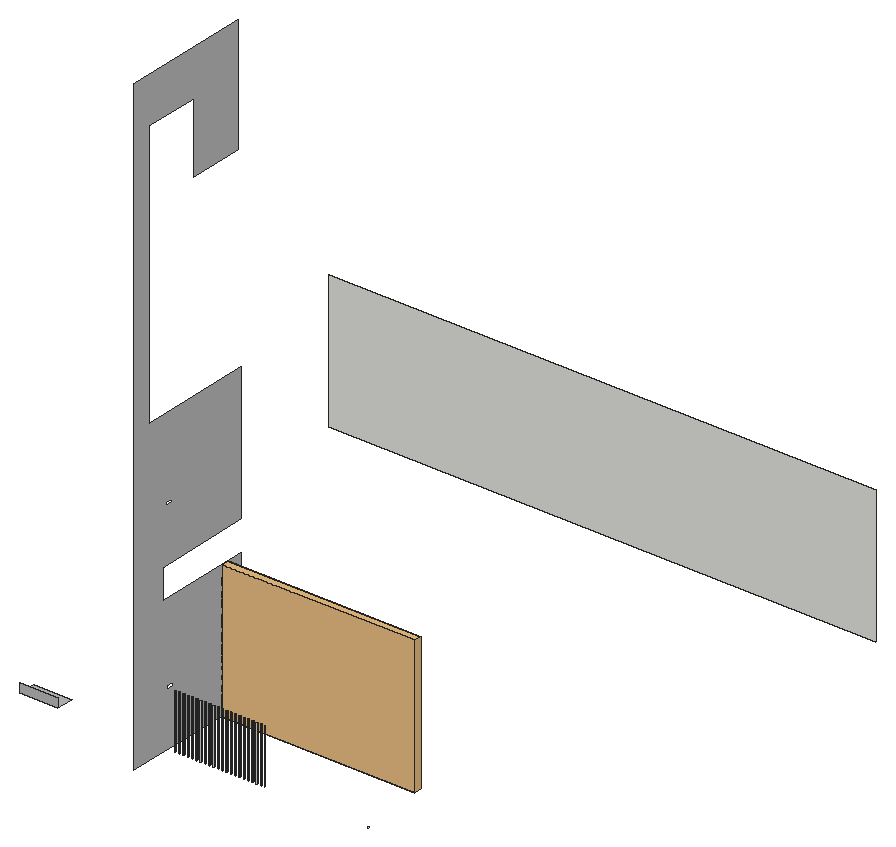
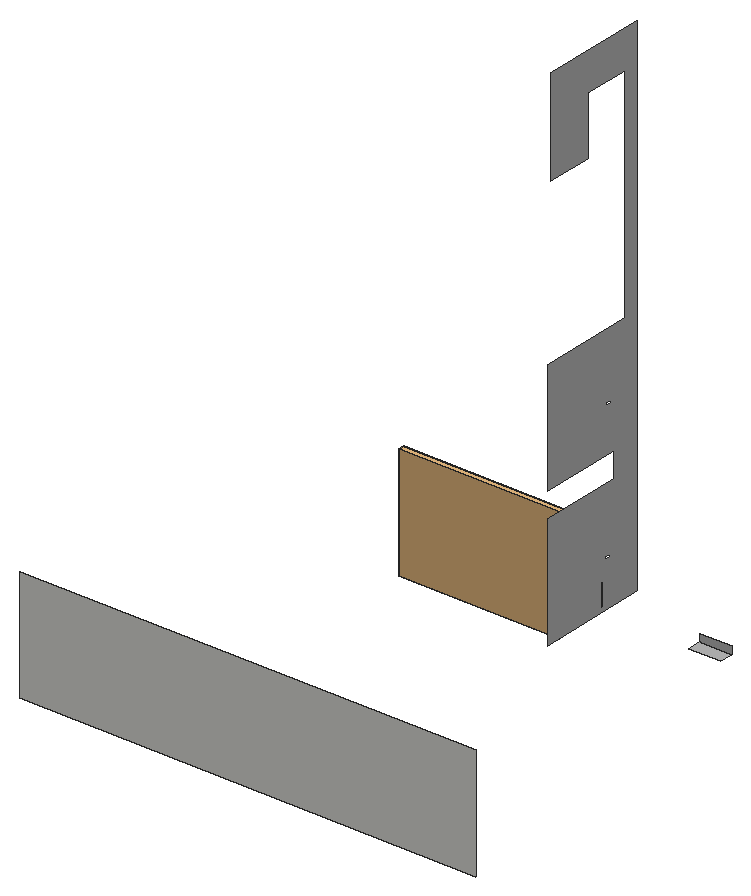
# SketchUp Ruby script. Lengths in inches.
U = 1.inch
M = Sketchup.active_model
def pt(a) = Geom::Point3d.new(a.map { |v| v * U })
def face(e, loops, mat)
  f = e.add_face(loops[0].map { |a| pt(a) })
  loops[1..].each { |l| e.add_face(l.map { |a| pt(a) }).erase! }
  f.material = f.back_material = mat if mat
  f
end
# faces: each face lists its corners as indices into pts; further lists are holes
def faces(e, pts, list, mat = nil) = list.each { |f| face(e, (f[0].is_a?(Array) ? f : [f]).map { |l| l.map { |i| pts[i] } }, mat) }
# xy, xz, yz: faces in a plane at the given z, y or x. An outline is a flat list of corners, or four numbers for a rectangle; further outlines are holes
def ring(l) = l.size == 4 ? [[l[0], l[1]], [l[2], l[1]], [l[2], l[3]], [l[0], l[3]]] : l.each_slice(2).to_a
def flat(e, list, mat, &to3) = list.each { |f| face(e, (f[0].is_a?(Array) ? f : [f]).map { |l| ring(l).map { |u, v| to3.(u, v) } }, mat) }
def xy(e, z, list, mat = nil) = flat(e, list, mat) { |x, y| [x, y, z] }
def xz(e, y, list, mat = nil) = flat(e, list, mat) { |x, z| [x, y, z] }
def yz(e, x, list, mat = nil) = flat(e, list, mat) { |y, z| [x, y, z] }
def lines(e, pts, list) = list.each { |a, b| e.add_line(pt(pts[a]), pt(pts[b])) }
# prism: a flat outline (further loops are holes) pulled along v
def prism(e, loops, v, mat = nil)
  f = face(e, loops, mat); d = Geom::Vector3d.new(v.map { |x| x * U })
  f.pushpull(f.normal.samedirection?(d) ? d.length : -d.length)
end
def box(e, o, s, mat = nil) = prism(e, [[o, [o[0] + s[0], o[1], o[2]], [o[0] + s[0], o[1] + s[1], o[2]], [o[0], o[1] + s[1], o[2]]]], [0, 0, s[2]], mat)
def at(x, y, z, deg = 0) = Geom::Transformation.translation(pt([x, y, z])) * Geom::Transformation.rotation(ORIGIN, Z_AXIS, deg.degrees)
def axes(o, x, y, z) = Geom::Transformation.new([*x, 0, *y, 0, *z, 0, *pt(o).to_a, 1])
def part(name) = M.definitions.add(name)
# library, detail: a bought-in or finely detailed component or shape, given as its bounding box
def library(name, o, s) = part(name).tap { |d| box(d.entities, o, s) }
def detail(e, o, s) = box(e.add_group.entities, o, s)
def put(e, d, t, mat = nil) = e.add_instance(d, t).tap { |i| i.material = mat if mat }
def group(e, t, mat = nil) = e.add_group.tap { |g| g.transformation = t; g.material = mat if mat }.entities
root = M.entities
M.materials.add("Generic\#2").color = [186, 186, 186]
c1 = part("Group\#1")
xy(c1.entities,0,[[0,0,46.77,20.375]])
xz(c1.entities,0,[[0,0,46.77,11.0625]])
c2 = library("Group\#9",[0,0,0],[238.3125,8.75,168])
xy(root,409.875,[[536.42,133.41,536.21,133.44,536.01,133.52,535.84,133.65,535.71,133.82,535.63,134.02,535.61,134.23,535.63,134.4375,535.71,134.63,535.84,134.8,536.01,134.93,536.21,135.01,536.42,135.04,536.63,135.01,536.82,134.93,536.99,134.8,537.12,134.63,537.2,134.4375,537.23,134.23,537.2,134.02,537.12,133.82,536.99,133.65,536.82,133.52,536.63,133.44]])
xz(root,724.5,[[15.3125,409.875,690.4375,577.875]])
yz(root,290.4375,[[[81.125,409.875,246,409.875,246,577.875,124.5,577.875,124.5,614.8125,246,614.8125,246,782.8125,103.5,782.8125,103.5,1111.375,172.5,1111.375,172.5,1024.6875,241.25,1024.6875,241.25,1168.125,81.125,1168.125],[129.43,680.58,138.74,684.77],[131.37,477.08,140.67,481.27]]],"Generic\#2")
p = [[297.51,134.4375,409.875],[297.48,134.23,409.875],[297.48,134.23,477.08],[297.51,134.4375,477.08],[299.11,134.23,409.875],[299.08,134.4375,409.875],
  [299.08,134.4375,477.08],[299.11,134.23,477.08],[302.82,134.4375,409.875],[302.79,134.23,409.875],[302.79,134.23,477.08],[302.82,134.4375,477.08],
  [304.42,134.23,409.875],[304.39,134.4375,409.875],[304.39,134.4375,477.08],[304.42,134.23,477.08],[308.13,134.4375,409.875],[308.11,134.23,409.875],
  [308.11,134.23,477.08],[308.13,134.4375,477.08],[309.73,134.23,409.875],[309.7,134.4375,409.875],[309.7,134.4375,477.08],[309.73,134.23,477.08],
  [313.45,134.4375,409.875],[313.42,134.23,409.875],[313.42,134.23,477.08],[313.45,134.4375,477.08],[315.04,134.23,409.875],[315.02,134.4375,409.875],
  [315.02,134.4375,477.08],[315.04,134.23,477.08],[318.76,134.4375,409.875],[318.73,134.23,409.875],[318.73,134.23,477.08],[318.76,134.4375,477.08],
  [320.36,134.23,409.875],[320.33,134.4375,409.875],[320.33,134.4375,477.08],[320.36,134.23,477.08],[324.07,134.4375,409.875],[324.04,134.23,409.875],
  [324.04,134.23,477.08],[324.07,134.4375,477.08],[325.67,134.23,409.875],[325.64,134.4375,409.875],[325.64,134.4375,477.08],[325.67,134.23,477.08],
  [329.38,134.4375,409.875],[329.36,134.23,409.875],[329.36,134.23,477.08],[329.38,134.4375,477.08],[330.98,134.23,409.875],[330.95,134.4375,409.875],
  [330.95,134.4375,477.08],[330.98,134.23,477.08],[334.7,134.4375,409.875],[334.67,134.23,409.875],[334.67,134.23,477.08],[334.7,134.4375,477.08],
  [336.29,134.23,409.875],[336.27,134.4375,409.875],[336.27,134.4375,477.08],[336.29,134.23,477.08],[340.01,134.4375,409.875],[339.98,134.23,409.875],
  [339.98,134.23,477.08],[340.01,134.4375,477.08],[341.61,134.23,409.875],[341.58,134.4375,409.875],[341.58,134.4375,477.08],[341.61,134.23,477.08],
  [345.32,134.4375,409.875],[345.29,134.23,409.875],[345.29,134.23,477.08],[345.32,134.4375,477.08],[346.92,134.23,409.875],[346.89,134.4375,409.875],
  [346.89,134.4375,477.08],[346.92,134.23,477.08],[350.63,134.4375,409.875],[350.61,134.23,409.875],[350.61,134.23,477.08],[350.63,134.4375,477.08],
  [352.23,134.23,409.875],[352.2,134.4375,409.875],[352.2,134.4375,477.08],[352.23,134.23,477.08],[355.95,134.4375,409.875],[355.92,134.23,409.875],
  [355.92,134.23,477.08],[355.95,134.4375,477.08],[357.54,134.23,409.875],[357.52,134.4375,409.875],[357.52,134.4375,477.08],[357.54,134.23,477.08],
  [361.26,134.4375,409.875],[361.23,134.23,409.875],[361.23,134.23,477.08],[361.26,134.4375,477.08],[362.86,134.23,409.875],[362.83,134.4375,409.875],
  [362.83,134.4375,477.08],[362.86,134.23,477.08],[366.57,134.4375,409.875],[366.54,134.23,409.875],[366.54,134.23,477.08],[366.57,134.4375,477.08],
  [368.17,134.23,409.875],[368.14,134.4375,409.875],[368.14,134.4375,477.08],[368.17,134.23,477.08],[371.88,134.4375,409.875],[371.86,134.23,409.875],
  [371.86,134.23,477.08],[371.88,134.4375,477.08],[373.48,134.23,409.875],[373.45,134.4375,409.875],[373.45,134.4375,477.08],[373.48,134.23,477.08],
  [377.2,134.4375,409.875],[377.17,134.23,409.875],[377.17,134.23,477.08],[377.2,134.4375,477.08],[378.79,134.23,409.875],[378.77,134.4375,409.875],
  [378.77,134.4375,477.08],[378.79,134.23,477.08],[382.51,134.4375,409.875],[382.48,134.23,409.875],[382.48,134.23,477.08],[382.51,134.4375,477.08],
  [384.11,134.23,409.875],[384.08,134.4375,409.875],[384.08,134.4375,477.08],[384.11,134.23,477.08],[387.82,134.4375,409.875],[387.79,134.23,409.875],
  [387.79,134.23,477.08],[387.82,134.4375,477.08],[389.42,134.23,409.875],[389.39,134.4375,409.875],[389.39,134.4375,477.08],[389.42,134.23,477.08],
  [393.13,134.4375,409.875],[393.11,134.23,409.875],[393.11,134.23,477.08],[393.13,134.4375,477.08],[394.73,134.23,409.875],[394.7,134.4375,409.875],
  [394.7,134.4375,477.08],[394.73,134.23,477.08],[398.45,134.4375,409.875],[398.42,134.23,409.875],[398.42,134.23,477.08],[398.45,134.4375,477.08],
  [400.04,134.23,409.875],[400.02,134.4375,409.875],[400.02,134.4375,477.08],[400.04,134.23,477.08],[403.76,134.4375,409.875],[403.73,134.23,409.875],
  [403.73,134.23,477.08],[403.76,134.4375,477.08],[405.36,134.23,409.875],[405.33,134.4375,409.875],[405.33,134.4375,477.08],[405.36,134.23,477.08],
  [409.07,134.4375,409.875],[409.04,134.23,409.875],[409.04,134.23,477.08],[409.07,134.4375,477.08],[297.59,134.63,409.875],[297.59,134.63,477.08],
  [299,134.63,409.875],[299,134.63,477.08],[302.9,134.63,409.875],[302.9,134.63,477.08],[304.31,134.63,409.875],[304.31,134.63,477.08],
  [308.21,134.63,409.875],[308.21,134.63,477.08],[309.62,134.63,409.875],[309.62,134.63,477.08],[313.53,134.63,409.875],[313.53,134.63,477.08],
  [314.93,134.63,409.875],[314.93,134.63,477.08],[318.84,134.63,409.875],[318.84,134.63,477.08],[320.25,134.63,409.875],[320.25,134.63,477.08],
  [324.15,134.63,409.875],[324.15,134.63,477.08],[325.56,134.63,409.875],[325.56,134.63,477.08],[329.46,134.63,409.875],[329.46,134.63,477.08],
  [330.87,134.63,409.875],[330.87,134.63,477.08],[334.78,134.63,409.875],[334.78,134.63,477.08],[336.18,134.63,409.875],[336.18,134.63,477.08],
  [340.09,134.63,409.875],[340.09,134.63,477.08],[341.5,134.63,409.875],[341.5,134.63,477.08],[345.4,134.63,409.875],[345.4,134.63,477.08],
  [346.81,134.63,409.875],[346.81,134.63,477.08],[350.71,134.63,409.875],[350.71,134.63,477.08],[352.12,134.63,409.875],[352.12,134.63,477.08],
  [356.03,134.63,409.875],[356.03,134.63,477.08],[357.43,134.63,409.875],[357.43,134.63,477.08],[361.34,134.63,409.875],[361.34,134.63,477.08],
  [362.75,134.63,409.875],[362.75,134.63,477.08],[366.65,134.63,409.875],[366.65,134.63,477.08],[368.06,134.63,409.875],[368.06,134.63,477.08],
  [371.96,134.63,409.875],[371.96,134.63,477.08],[373.37,134.63,409.875],[373.37,134.63,477.08],[377.28,134.63,409.875],[377.28,134.63,477.08],
  [378.68,134.63,409.875],[378.68,134.63,477.08],[382.59,134.63,409.875],[382.59,134.63,477.08],[384,134.63,409.875],[384,134.63,477.08],
  [387.9,134.63,409.875],[387.9,134.63,477.08],[389.31,134.63,409.875],[389.31,134.63,477.08],[393.21,134.63,409.875],[393.21,134.63,477.08],
  [394.62,134.63,409.875],[394.62,134.63,477.08],[398.53,134.63,409.875],[398.53,134.63,477.08],[399.93,134.63,409.875],[399.93,134.63,477.08],
  [403.84,134.63,409.875],[403.84,134.63,477.08],[405.25,134.63,409.875],[405.25,134.63,477.08],[409.15,134.63,409.875],[409.15,134.63,477.08],
  [297.72,134.8,409.875],[297.72,134.8,477.08],[298.87,134.8,409.875],[298.87,134.8,477.08],[303.03,134.8,409.875],[303.03,134.8,477.08],
  [304.18,134.8,409.875],[304.18,134.8,477.08],[308.34,134.8,409.875],[308.34,134.8,477.08],[309.49,134.8,409.875],[309.49,134.8,477.08],
  [313.66,134.8,409.875],[313.66,134.8,477.08],[314.8,134.8,409.875],[314.8,134.8,477.08],[318.97,134.8,409.875],[318.97,134.8,477.08],
  [320.12,134.8,409.875],[320.12,134.8,477.08],[324.28,134.8,409.875],[324.28,134.8,477.08],[325.43,134.8,409.875],[325.43,134.8,477.08],
  [329.59,134.8,409.875],[329.59,134.8,477.08],[330.74,134.8,409.875],[330.74,134.8,477.08],[334.91,134.8,409.875],[334.91,134.8,477.08],
  [336.05,134.8,409.875],[336.05,134.8,477.08],[340.22,134.8,409.875],[340.22,134.8,477.08],[341.37,134.8,409.875],[341.37,134.8,477.08],
  [345.53,134.8,409.875],[345.53,134.8,477.08],[346.68,134.8,409.875],[346.68,134.8,477.08],[350.84,134.8,409.875],[350.84,134.8,477.08],
  [351.99,134.8,409.875],[351.99,134.8,477.08],[356.16,134.8,409.875],[356.16,134.8,477.08],[357.3,134.8,409.875],[357.3,134.8,477.08],
  [361.47,134.8,409.875],[361.47,134.8,477.08],[362.62,134.8,409.875],[362.62,134.8,477.08],[366.78,134.8,409.875],[366.78,134.8,477.08],
  [367.93,134.8,409.875],[367.93,134.8,477.08],[372.09,134.8,409.875],[372.09,134.8,477.08],[373.24,134.8,409.875],[373.24,134.8,477.08],
  [377.41,134.8,409.875],[377.41,134.8,477.08],[378.55,134.8,409.875],[378.55,134.8,477.08],[382.72,134.8,409.875],[382.72,134.8,477.08],
  [383.87,134.8,409.875],[383.87,134.8,477.08],[388.03,134.8,409.875],[388.03,134.8,477.08],[389.18,134.8,409.875],[389.18,134.8,477.08],
  [393.34,134.8,409.875],[393.34,134.8,477.08],[394.49,134.8,409.875],[394.49,134.8,477.08],[398.66,134.8,409.875],[398.66,134.8,477.08],
  [399.8,134.8,409.875],[399.8,134.8,477.08],[403.97,134.8,409.875],[403.97,134.8,477.08],[405.12,134.8,409.875],[405.12,134.8,477.08],
  [297.89,134.93,409.875],[297.89,134.93,477.08],[298.7,134.93,409.875],[298.7,134.93,477.08],[303.2,134.93,409.875],[303.2,134.93,477.08],
  [304.01,134.93,409.875],[304.01,134.93,477.08],[308.51,134.93,409.875],[308.51,134.93,477.08],[309.32,134.93,409.875],[309.32,134.93,477.08],
  [313.82,134.93,409.875],[313.82,134.93,477.08],[314.64,134.93,409.875],[314.64,134.93,477.08],[319.14,134.93,409.875],[319.14,134.93,477.08],
  [319.95,134.93,409.875],[319.95,134.93,477.08],[324.45,134.93,409.875],[324.45,134.93,477.08],[325.26,134.93,409.875],[325.26,134.93,477.08],
  [329.76,134.93,409.875],[329.76,134.93,477.08],[330.57,134.93,409.875],[330.57,134.93,477.08],[335.07,134.93,409.875],[335.07,134.93,477.08],
  [335.89,134.93,409.875],[335.89,134.93,477.08],[340.39,134.93,409.875],[340.39,134.93,477.08],[341.2,134.93,409.875],[341.2,134.93,477.08],
  [345.7,134.93,409.875],[345.7,134.93,477.08],[346.51,134.93,409.875],[346.51,134.93,477.08],[351.01,134.93,409.875],[351.01,134.93,477.08],
  [351.82,134.93,409.875],[351.82,134.93,477.08],[356.32,134.93,409.875],[356.32,134.93,477.08],[357.14,134.93,409.875],[357.14,134.93,477.08],
  [361.64,134.93,409.875],[361.64,134.93,477.08],[362.45,134.93,409.875],[362.45,134.93,477.08],[366.95,134.93,409.875],[366.95,134.93,477.08],
  [367.76,134.93,409.875],[367.76,134.93,477.08],[372.26,134.93,409.875],[372.26,134.93,477.08],[373.07,134.93,409.875],[373.07,134.93,477.08],
  [377.57,134.93,409.875],[377.57,134.93,477.08],[378.39,134.93,409.875],[378.39,134.93,477.08],[382.89,134.93,409.875],[382.89,134.93,477.08],
  [383.7,134.93,409.875],[383.7,134.93,477.08],[388.2,134.93,409.875],[388.2,134.93,477.08],[389.01,134.93,409.875],[389.01,134.93,477.08],
  [393.51,134.93,409.875],[393.51,134.93,477.08],[394.32,134.93,409.875],[394.32,134.93,477.08],[398.82,134.93,409.875],[398.82,134.93,477.08],
  [399.64,134.93,409.875],[399.64,134.93,477.08],[404.14,134.93,409.875],[404.14,134.93,477.08],[404.95,134.93,409.875],[404.95,134.93,477.08],
  [298.08,135.01,409.875],[298.08,135.01,477.08],[298.5,135.01,409.875],[298.5,135.01,477.08],[303.4,135.01,409.875],[303.4,135.01,477.08],
  [303.82,135.01,409.875],[303.82,135.01,477.08],[308.71,135.01,409.875],[308.71,135.01,477.08],[309.13,135.01,409.875],[309.13,135.01,477.08],
  [314.02,135.01,409.875],[314.02,135.01,477.08],[314.44,135.01,409.875],[314.44,135.01,477.08],[319.33,135.01,409.875],[319.33,135.01,477.08],
  [319.75,135.01,409.875],[319.75,135.01,477.08],[324.65,135.01,409.875],[324.65,135.01,477.08],[325.07,135.01,409.875],[325.07,135.01,477.08],
  [329.96,135.01,409.875],[329.96,135.01,477.08],[330.38,135.01,409.875],[330.38,135.01,477.08],[335.27,135.01,409.875],[335.27,135.01,477.08],
  [335.69,135.01,409.875],[335.69,135.01,477.08],[340.58,135.01,409.875],[340.58,135.01,477.08],[341,135.01,409.875],[341,135.01,477.08],
  [345.9,135.01,409.875],[345.9,135.01,477.08],[346.32,135.01,409.875],[346.32,135.01,477.08],[351.21,135.01,409.875],[351.21,135.01,477.08],
  [351.63,135.01,409.875],[351.63,135.01,477.08],[356.52,135.01,409.875],[356.52,135.01,477.08],[356.94,135.01,409.875],[356.94,135.01,477.08],
  [361.83,135.01,409.875],[361.83,135.01,477.08],[362.25,135.01,409.875],[362.25,135.01,477.08],[367.15,135.01,409.875],[367.15,135.01,477.08],
  [367.57,135.01,409.875],[367.57,135.01,477.08],[372.46,135.01,409.875],[372.46,135.01,477.08],[372.88,135.01,409.875],[372.88,135.01,477.08],
  [377.77,135.01,409.875],[377.77,135.01,477.08],[378.19,135.01,409.875],[378.19,135.01,477.08],[383.08,135.01,409.875],[383.08,135.01,477.08],
  [383.5,135.01,409.875],[383.5,135.01,477.08],[388.4,135.01,409.875],[388.4,135.01,477.08],[388.82,135.01,409.875],[388.82,135.01,477.08],
  [393.71,135.01,409.875],[393.71,135.01,477.08],[394.13,135.01,409.875],[394.13,135.01,477.08],[399.02,135.01,409.875],[399.02,135.01,477.08],
  [399.44,135.01,409.875],[399.44,135.01,477.08],[404.33,135.01,409.875],[404.33,135.01,477.08],[404.75,135.01,409.875],[404.75,135.01,477.08],
  [298.29,135.04,409.875],[298.29,135.04,477.08],[303.61,135.04,409.875],[303.61,135.04,477.08],[308.92,135.04,409.875],[308.92,135.04,477.08],
  [314.23,135.04,409.875],[314.23,135.04,477.08],[319.54,135.04,409.875],[319.54,135.04,477.08],[324.86,135.04,409.875],[324.86,135.04,477.08],
  [330.17,135.04,409.875],[330.17,135.04,477.08],[335.48,135.04,409.875],[335.48,135.04,477.08],[340.79,135.04,409.875],[340.79,135.04,477.08],
  [346.11,135.04,409.875],[346.11,135.04,477.08],[351.42,135.04,409.875],[351.42,135.04,477.08],[356.73,135.04,409.875],[356.73,135.04,477.08],
  [362.04,135.04,409.875],[362.04,135.04,477.08],[367.36,135.04,409.875],[367.36,135.04,477.08],[372.67,135.04,409.875],[372.67,135.04,477.08],
  [377.98,135.04,409.875],[377.98,135.04,477.08],[383.29,135.04,409.875],[383.29,135.04,477.08],[388.61,135.04,409.875],[388.61,135.04,477.08],
  [393.92,135.04,409.875],[393.92,135.04,477.08],[399.23,135.04,409.875],[399.23,135.04,477.08],[404.54,135.04,409.875],[404.54,135.04,477.08]]
faces(root,p,[[0,1,2,3],[4,5,6,7],[8,9,10,11],[12,13,14,15],[16,17,18,19],[20,21,22,23],[24,25,26,27],[28,29,30,31],
  [32,33,34,35],[36,37,38,39],[40,41,42,43],[44,45,46,47],[48,49,50,51],[52,53,54,55],[56,57,58,59],[60,61,62,63],
  [64,65,66,67],[68,69,70,71],[72,73,74,75],[76,77,78,79],[80,81,82,83],[84,85,86,87],[88,89,90,91],[92,93,94,95],
  [96,97,98,99],[100,101,102,103],[104,105,106,107],[108,109,110,111],[112,113,114,115],[116,117,118,119],[120,121,122,123],[124,125,126,127],
  [128,129,130,131],[132,133,134,135],[136,137,138,139],[140,141,142,143],[144,145,146,147],[148,149,150,151],[152,153,154,155],[156,157,158,159],
  [160,161,162,163],[164,165,166,167],[168,169,170,171],[172,0,3,173],[5,174,175,6],[176,8,11,177],[13,178,179,14],[180,16,19,181],
  [21,182,183,22],[184,24,27,185],[29,186,187,30],[188,32,35,189],[37,190,191,38],[192,40,43,193],[45,194,195,46],[196,48,51,197],
  [53,198,199,54],[200,56,59,201],[61,202,203,62],[204,64,67,205],[69,206,207,70],[208,72,75,209],[77,210,211,78],[212,80,83,213],
  [85,214,215,86],[216,88,91,217],[93,218,219,94],[220,96,99,221],[101,222,223,102],[224,104,107,225],[109,226,227,110],[228,112,115,229],
  [117,230,231,118],[232,120,123,233],[125,234,235,126],[236,128,131,237],[133,238,239,134],[240,136,139,241],[141,242,243,142],[244,144,147,245],
  [149,246,247,150],[248,152,155,249],[157,250,251,158],[252,160,163,253],[165,254,255,166],[256,168,171,257],[258,172,173,259],[174,260,261,175],
  [262,176,177,263],[178,264,265,179],[266,180,181,267],[182,268,269,183],[270,184,185,271],[186,272,273,187],[274,188,189,275],[190,276,277,191],
  [278,192,193,279],[194,280,281,195],[282,196,197,283],[198,284,285,199],[286,200,201,287],[202,288,289,203],[290,204,205,291],[206,292,293,207],
  [294,208,209,295],[210,296,297,211],[298,212,213,299],[214,300,301,215],[302,216,217,303],[218,304,305,219],[306,220,221,307],[222,308,309,223],
  [310,224,225,311],[226,312,313,227],[314,228,229,315],[230,316,317,231],[318,232,233,319],[234,320,321,235],[322,236,237,323],[238,324,325,239],
  [326,240,241,327],[242,328,329,243],[330,244,245,331],[246,332,333,247],[334,248,249,335],[250,336,337,251],[338,252,253,339],[254,340,341,255],
  [342,258,259,343],[260,344,345,261],[346,262,263,347],[264,348,349,265],[350,266,267,351],[268,352,353,269],[354,270,271,355],[272,356,357,273],
  [358,274,275,359],[276,360,361,277],[362,278,279,363],[280,364,365,281],[366,282,283,367],[284,368,369,285],[370,286,287,371],[288,372,373,289],
  [374,290,291,375],[292,376,377,293],[378,294,295,379],[296,380,381,297],[382,298,299,383],[300,384,385,301],[386,302,303,387],[304,388,389,305],
  [390,306,307,391],[308,392,393,309],[394,310,311,395],[312,396,397,313],[398,314,315,399],[316,400,401,317],[402,318,319,403],[320,404,405,321],
  [406,322,323,407],[324,408,409,325],[410,326,327,411],[328,412,413,329],[414,330,331,415],[332,416,417,333],[418,334,335,419],[336,420,421,337],
  [422,338,339,423],[340,424,425,341],[426,342,343,427],[344,428,429,345],[430,346,347,431],[348,432,433,349],[434,350,351,435],[352,436,437,353],
  [438,354,355,439],[356,440,441,357],[442,358,359,443],[360,444,445,361],[446,362,363,447],[364,448,449,365],[450,366,367,451],[368,452,453,369],
  [454,370,371,455],[372,456,457,373],[458,374,375,459],[376,460,461,377],[462,378,379,463],[380,464,465,381],[466,382,383,467],[384,468,469,385],
  [470,386,387,471],[388,472,473,389],[474,390,391,475],[392,476,477,393],[478,394,395,479],[396,480,481,397],[482,398,399,483],[400,484,485,401],
  [486,402,403,487],[404,488,489,405],[490,406,407,491],[408,492,493,409],[494,410,411,495],[412,496,497,413],[498,414,415,499],[416,500,501,417],
  [502,418,419,503],[420,504,505,421],[506,422,423,507],[424,508,509,425],[510,426,427,511],[428,510,511,429],[512,430,431,513],[432,512,513,433],
  [514,434,435,515],[436,514,515,437],[516,438,439,517],[440,516,517,441],[518,442,443,519],[444,518,519,445],[520,446,447,521],[448,520,521,449],
  [522,450,451,523],[452,522,523,453],[524,454,455,525],[456,524,525,457],[526,458,459,527],[460,526,527,461],[528,462,463,529],[464,528,529,465],
  [530,466,467,531],[468,530,531,469],[532,470,471,533],[472,532,533,473],[534,474,475,535],[476,534,535,477],[536,478,479,537],[480,536,537,481],
  [538,482,483,539],[484,538,539,485],[540,486,487,541],[488,540,541,489],[542,490,491,543],[492,542,543,493],[544,494,495,545],[496,544,545,497],
  [546,498,499,547],[500,546,547,501],[548,502,503,549],[504,548,549,505],[550,506,507,551],[508,550,551,509]])
put(root,c1,at(110.7,130.3125,410.125),"Generic\#2")
put(root,c2,at(290.4375,216.0625,409.875))
